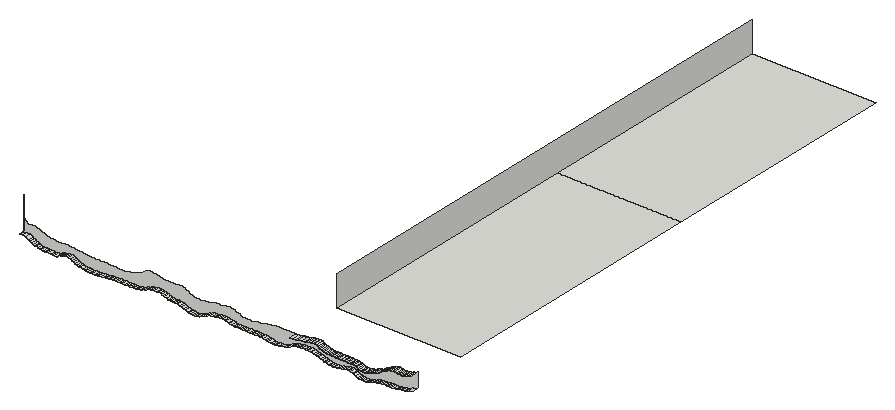
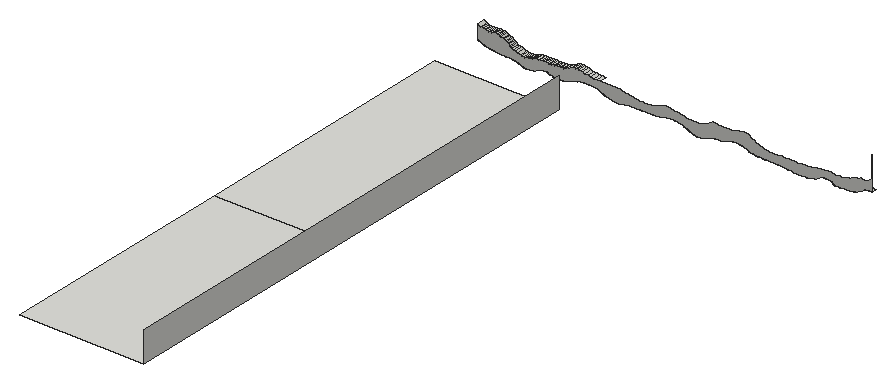
# SketchUp Ruby script. Lengths in inches.
U = 1.inch
M = Sketchup.active_model
def pt(a) = Geom::Point3d.new(a.map { |v| v * U })
def face(e, loops, mat)
  f = e.add_face(loops[0].map { |a| pt(a) })
  loops[1..].each { |l| e.add_face(l.map { |a| pt(a) }).erase! }
  f.material = f.back_material = mat if mat
  f
end
# faces: each face lists its corners as indices into pts; further lists are holes
def faces(e, pts, list, mat = nil) = list.each { |f| face(e, (f[0].is_a?(Array) ? f : [f]).map { |l| l.map { |i| pts[i] } }, mat) }
# xy, xz, yz: faces in a plane at the given z, y or x. An outline is a flat list of corners, or four numbers for a rectangle; further outlines are holes
def ring(l) = l.size == 4 ? [[l[0], l[1]], [l[2], l[1]], [l[2], l[3]], [l[0], l[3]]] : l.each_slice(2).to_a
def flat(e, list, mat, &to3) = list.each { |f| face(e, (f[0].is_a?(Array) ? f : [f]).map { |l| ring(l).map { |u, v| to3.(u, v) } }, mat) }
def xy(e, z, list, mat = nil) = flat(e, list, mat) { |x, y| [x, y, z] }
def xz(e, y, list, mat = nil) = flat(e, list, mat) { |x, z| [x, y, z] }
def yz(e, x, list, mat = nil) = flat(e, list, mat) { |y, z| [x, y, z] }
def lines(e, pts, list) = list.each { |a, b| e.add_line(pt(pts[a]), pt(pts[b])) }
# prism: a flat outline (further loops are holes) pulled along v
def prism(e, loops, v, mat = nil)
  f = face(e, loops, mat); d = Geom::Vector3d.new(v.map { |x| x * U })
  f.pushpull(f.normal.samedirection?(d) ? d.length : -d.length)
end
def box(e, o, s, mat = nil) = prism(e, [[o, [o[0] + s[0], o[1], o[2]], [o[0] + s[0], o[1] + s[1], o[2]], [o[0], o[1] + s[1], o[2]]]], [0, 0, s[2]], mat)
def at(x, y, z, deg = 0) = Geom::Transformation.translation(pt([x, y, z])) * Geom::Transformation.rotation(ORIGIN, Z_AXIS, deg.degrees)
def axes(o, x, y, z) = Geom::Transformation.new([*x, 0, *y, 0, *z, 0, *pt(o).to_a, 1])
def part(name) = M.definitions.add(name)
# library, detail: a bought-in or finely detailed component or shape, given as its bounding box
def library(name, o, s) = part(name).tap { |d| box(d.entities, o, s) }
def detail(e, o, s) = box(e.add_group.entities, o, s)
def put(e, d, t, mat = nil) = e.add_instance(d, t).tap { |i| i.material = mat if mat }
def group(e, t, mat = nil) = e.add_group.tap { |g| g.transformation = t; g.material = mat if mat }.entities
root = M.entities
xy(root,237.65,[[1160.83,2402.3,1161.52,2404.3],[1161.52,2402.3,1162.14,2404.3]])
xy(root,238.18,[[1254.78,2402.3,1255.46,2404.3]])
xy(root,238.33,[[1169.93,2402.3,1170.48,2404.3],[1170.48,2402.3,1171.16,2404.3]])
xy(root,238.34,[[1171.84,2402.3,1172.77,2404.3],[1172.77,2402.3,1173.26,2404.3],[1173.26,2402.3,1174.02,2404.3],[1174.02,2402.3,1174.65,2404.3],[1174.65,2402.3,1175.4,2404.3],
  [1175.4,2402.3,1176.02,2404.3],[1176.02,2402.3,1176.79,2404.3],[1176.79,2402.3,1177.41,2404.3]])
xy(root,238.62,[[1221.31,2402.3,1222.08,2404.3],[1222.08,2402.3,1222.71,2404.3],[1222.71,2402.3,1223.47,2404.3],[1223.47,2402.3,1224.09,2404.3],[1224.09,2402.3,1224.94,2404.3],
  [1224.94,2402.3,1225.58,2404.3],[1225.58,2402.3,1226.2,2404.3]])
xy(root,238.625,[[1219.89,2402.3,1220.75,2404.3]])
xy(root,238.89,[[1275.7,2402.3,1276.38,2404.3]])
xy(root,238.9,[[1277.14,2402.3,1277.76,2404.3],[1277.76,2402.3,1278.53,2404.3]])
xy(root,240.43,[[1243.98,2402.3,1244.55,2404.3]])
xy(root,241.52,[[1131.53,2402.3,1131.59,2404.3]])
xy(root,242.28,[[1261.8,2401.37,1262.3125,2404.3]])
xy(root,242.3,[[1260.04,2401.37,1260.71,2404.3]])
xy(root,242.33,[[1257.63,2401.37,1258.21,2404.3]])
xy(root,242.625,[[1237.14,2425.46,1285.6,2532.83],[1237.14,2532.83,1285.6,2628.15]])
xz(root,2404.3,[[1200.45,236.98,1199.84,237.01,1199.15,237.04,1198.39,237.11,1197.7,237.2,1197.17,237.33,1196.5,237.68,1195.5625,237.96,1195,238.28,1194.22,238.43,1193.44,238.78,1192.77,238.79,1192.23,238.8,1191.47,238.83,1190.72,238.875,1190.15,238.94,1189.57,239.04,1188.91,239.29,1188.33,239.53,1187.8,239.7,1187.11,239.92,1186.48,240.11,1185.7,240.27,1185.08,240.25,1184.375,240.23,1183.61,240.19,1182.9375,240.12,1182.28,240.03,1181.64,239.85,1181.09,239.52,1180.53,239.35,1179.94,239.18,1179.43,238.86,1178.74,238.72,1177.92,238.59,1177.41,238.34,1171.84,238.34,1171.16,238.33,1169.93,238.33,1169.21,238.32,1168.36,238.3,1167.73,238.28,1166.98,238.26,1166.35,238.15,1165.59,238.13,1165.04,238.1,1164.1875,237.98,1163.57,237.94,1162.81,237.89,1162.14,237.65,1160.83,237.65,1160.14,237.66,1159.39,237.67,1158.79,237.68,1158.18,237.71,1157.47,237.76,1156.78,237.82,1156.12,237.9,1155.18,238.21,1154.71,238.31,1153.8,238.43,1153.15,238.74,1152.57,239.11,1151.99,239.38,1151.53,239.71,1150.83,240.11,1150.14,240.09,1149.48,240.05,1148.89,239.99,1148.16,239.88,1147.61,239.69,1147.03,239.55,1146.47,238.9375,1145.94,238.77,1145.2,238.79,1144.33,238.8,1143.82,238.82,1142.78,238.92,1142.09,238.93,1141.39,238.94,1140.69,238.97,1140.01,239.03,1139.32,239.09,1138.54,239.19,1138.03,239.52,1137.47,239.64,1137.02,239.86,1136.23,240.2,1135.63,240.59,1135.09,240.85,1134.07,241.55,1132.8,241.69,1131.59,241.52,1131.59,246.2,1133.16,244.96,1134.55,244.9375,1135.8,244.92,1136.02,244.61,1136.58,244.54,1137.34,244.41,1138.01,244.11,1138.53,243.95,1139.19,243.79,1139.71,243.48,1140.35,243.3,1140.9375,243.14,1141.42,243.06,1142.14,242.85,1142.72,242.78,1143.53,242.73,1144.07,242.68,1144.74,242.51,1145.26,242.46,1145.8,242.58,1146.43,242.57,1147.06,242.81,1147.63,242.86,1148.19,242.89,1148.83,242.92,1149.26,242.625,1149.87,242.65,1150.42,242.62,1151.05,242.58,1151.61,242.57,1152.25,242.48,1152.91,242.38,1153.57,242.34,1154.24,242.24,1155.41,241.96,1156.18,241.89,1157,241.83,1157.6,241.78,1158.37,241.75,1158.82,241.74,1159.37,241.72,1160.63,241.7,1161.36,241.69,1162.03,241.68,1162.62,241.68,1163.11,241.67,1163.8125,241.74,1164.38,241.75,1166.38,241.75,1166.87,241.67,1167.4,241.66,1168.01,241.57,1168.55,241.53,1169.17,241.51,1169.72,241.49,1170.42,241.48,1171.08,241.47,1171.65,241.46,1172.36,241.6,1173.09,241.85,1173.76,241.91,1174.66,242.1,1175.43,242.46,1176.13,242.78,1176.9,242.97,1177.43,243.23,1177.83,243.48,1178.35,243.72,1178.6875,244.12,1179.16,244.39,1179.64,244.73,1180.125,244.87,1180.71,244.95,1181.39,245.01,1182.04,244.81,1182.61,244.7,1183.09,244.67,1183.7,244.55,1184.24,244.51,1184.7,244.25,1185.45,244.11,1186.01,244.04,1186.63,243.99,1187.35,243.95,1187.85,243.93,1188.54,243.91,1189.11,243.89,1189.81,243.88,1190.46,243.94,1191.1,243.95,1191.66,244.1,1192.29,244.13,1192.77,244.15,1193.29,244.17,1193.81,244.18,1194.41,243.8,1194.95,243.43,1195.56,243.09,1195.95,242.875,1196.45,242.68,1197.04,242.51,1197.55,242.21,1198.15,242.11,1198.83,241.96,1199.39,241.89,1199.85,241.85,1200.37,241.8125,1200.88,241.79,1201.46,241.78,1202.13,241.91,1202.6,241.93,1203.27,242.09,1204.04,242.2,1204.54,242.24,1205.15,242.42,1205.7,242.47,1206.45,242.71,1207.09,242.78,1207.57,242.82,1208.26,242.85,1208.96,242.87,1209.51,243.02,1210.13,243.05,1210.68,243.29,1211.36,243.35,1211.91,243.39,1212.51,243.42,1213.28,243.14,1213.85,242.9375,1214.4,242.65,1215.02,242.39,1215.78,242.14,1216.42,241.89,1216.91,241.78,1217.96,241.63,1218.73,241.56,1219.33,241.51,1219.78,241.48,1220.3,241.46,1221.17,241.51,1221.89,241.59,1222.83,241.82,1223.61,241.87,1224.375,241.98,1224.99,242.02,1225.64,242.19,1226.34,242.38,1226.83,242.4375,1227.35,242.48,1228.01,242.58,1228.54,242.61,1229.125,242.77,1229.58,242.95,1230.14,243.01,1230.65,243.05,1231.22,243.08,1231.875,243.09,1234.03,243.09,1234.6,243.08,1235.1875,243.07,1235.77,243.07,1236.43,243.0625,1237.04,243.05,1237.72,243.05,1238.99,243.1,1240.16,243.17,1241.3,243.4,1242.5625,243.52,1243.69,243.71,1244.59,243.99,1245.29,244.08,1245.99,244.21,1246.57,244.27,1247.11,244.3,1247.78,244.39,1248.375,244.19,1248.75,243.88,1249.23,243.59,1249.78,243.33,1250.33,243.22,1250.82,242.92,1251.3,242.75,1251.86,242.6,1252.42,242.52,1252.98,242.47,1253.5625,242.43,1254.14,242.4,1254.72,242.39,1255.3,242.37,1255.88,242.36,1256.47,242.35,1257.63,242.33,1258.21,242.33,1258.93,242.32,1259.4,242.3125,1260.04,242.3,1260.71,242.3,1261.16,242.29,1261.8,242.28,1262.3125,242.28,1262.94,242.2,1263.52,241.97,1264.09,241.84,1264.6,241.57,1265.02,241.33,1265.49,241.24,1266.02,241.17,1266.49,241.12,1267.09,241.09,1267.66,241.14,1268.3,241.35,1268.89,241.46,1269.83,241.85,1270.83,242.23,1271.39,242.42,1272.11,242.61,1272.625,242.91,1273,243.14,1273.54,243.52,1274.02,243.71,1274.35,244.02,1274.79,244.21,1275.38,244.57,1275.85,244.76,1276.47,245.125,1276.97,245.32,1277.45,245.41,1278,245.48,1278.49,245.59,1279.02,245.55,1279.63,245.35,1280.12,245.31,1280.67,245.27,1281.23,245.24,1281.79,245.22,1282.35,245.34,1282.98,245.42,1283.5625,245.52,1283.94,245.76,1284.41,245.9,1285.6,246.43,1285.6,240.89,1283.77,240.1,1283.21,239.96,1282.6875,239.81,1282,239.53,1281.45,239.49,1280.73,239.42,1279.93,239.28,1279.16,239.15,1278.53,238.9,1277.14,238.9,1276.38,238.89,1275.7,238.89,1275.02,238.88,1274.48,238.875,1273.72,238.86,1272.98,238.83,1272.41,238.8,1271.83,238.74,1271.17,238.6,1270.6,238.51,1270.07,238.33,1269.38,238.08,1268.7,237.84,1268.01,237.5625,1267.41,237.47,1266.73,237.4,1266,237.42,1265.43,237.45,1264.84,237.51,1264.24,237.59,1263.7,237.71,1262.87,238,1262.16,238.33,1261.61,238.57,1261.11,238.86,1260.59,238.96,1259.9,239.02,1259.22,239.125,1258.48,239.04,1257.91,238.66,1257.32,238.61,1256.66,238.55,1256.14,238.27,1255.46,238.18,1254.78,238.18,1254.11,238.11,1253.58,238.15,1252.76,238.19,1252.1875,238.26,1251.62,238.48,1250.96,238.56,1250.39,238.67,1249.87,239.01,1249.1875,239.18,1248.5625,239.5,1247.8,239.65,1247.1875,239.8,1246.43,239.96,1245.78,240.23,1245.2,240.27,1244.55,240.43,1243.98,240.43,1243.4,240.42,1242.875,240.41,1242.18,240.4,1241.49,240.37,1240.8,240.33,1240.12,240.27,1239.44,240.17,1238.82,239.97,1238.17,239.75,1237.43,239.375,1236.64,239.08,1235.76,238.72,1235.01,238.46,1233.79,238.14,1232.67,237.88,1232.02,237.87,1231.15,237.74,1230.44,237.79,1229.67,237.86,1229.04,238.15,1228.27,238.19,1227.65,238.25,1226.89,238.45,1226.2,238.62,1221.31,238.62,1220.75,238.625,1219.89,238.625,1219.2,238.63,1218.58,238.64,1217.8,238.65,1217.13,238.66,1216.44,238.6875,1215.77,238.73,1215.29,238.78,1214.41,238.93,1213.64,239.07,1213.09,239.16,1212.24,239.44,1211.57,239.56,1210.96,239.72,1210.23,239.7,1209.67,239.69,1209.08,239.65,1208.46,239.6,1207.97,239.54,1207.16,239.31,1206.16,239.22,1205.58,239.12,1204.9375,238.76,1204.3,238.51,1203.74,238.375,1203.3,238.02,1202.6,237.74,1201.98,237.43,1201.13,237.22],[1131.53,241.52,1131.59,254.5]])
yz(root,1237.14,[[2425.46,242.625,2628.15,254.5]])
p = [[1198.39,2404.3,237.11],[1199.15,2404.3,237.04],[1199.15,2402.3,237.04],[1198.39,2402.3,237.11],[1199.84,2404.3,237.01],[1199.84,2402.3,237.01],
  [1200.45,2404.3,236.98],[1200.45,2402.3,236.98],[1201.13,2404.3,237.22],[1201.13,2402.3,237.22],[1197.7,2404.3,237.2],[1197.7,2402.3,237.2],
  [1197.17,2404.3,237.33],[1197.17,2402.3,237.33],[1201.98,2404.3,237.43],[1201.98,2402.3,237.43],[1196.5,2404.3,237.68],[1196.5,2402.3,237.68],
  [1202.6,2404.3,237.74],[1202.6,2402.3,237.74],[1265.43,2404.3,237.45],[1266,2404.3,237.42],[1266,2402.3,237.42],[1265.43,2402.3,237.45],
  [1266.73,2404.3,237.4],[1266.73,2402.3,237.4],[1267.41,2404.3,237.47],[1267.41,2402.3,237.47],[1264.24,2404.3,237.59],[1264.84,2404.3,237.51],
  [1264.84,2402.3,237.51],[1264.24,2402.3,237.59],[1268.01,2404.3,237.5625],[1268.01,2402.3,237.5625],[1162.14,2404.3,237.65],[1162.81,2404.3,237.89],
  [1162.81,2402.3,237.89],[1162.14,2402.3,237.65],[1263.7,2404.3,237.71],[1263.7,2402.3,237.71],[1268.7,2404.3,237.84],[1268.7,2402.3,237.84],
  [1157.47,2404.3,237.76],[1158.18,2404.3,237.71],[1158.18,2402.3,237.71],[1157.47,2402.3,237.76],[1158.79,2404.3,237.68],[1158.79,2402.3,237.68],
  [1159.39,2404.3,237.67],[1159.39,2402.3,237.67],[1160.14,2404.3,237.66],[1160.14,2402.3,237.66],[1160.83,2404.3,237.65],[1160.83,2402.3,237.65],
  [1195.5625,2404.3,237.96],[1195.5625,2402.3,237.96],[1203.3,2404.3,238.02],[1203.3,2402.3,238.02],[1230.44,2404.3,237.79],[1231.15,2404.3,237.74],
  [1231.15,2402.3,237.74],[1230.44,2402.3,237.79],[1232.02,2404.3,237.87],[1232.02,2402.3,237.87],[1262.87,2404.3,238],[1262.87,2402.3,238],
  [1156.12,2404.3,237.9],[1156.78,2404.3,237.82],[1156.78,2402.3,237.82],[1156.12,2402.3,237.9],[1229.67,2404.3,237.86],[1229.67,2402.3,237.86],
  [1269.38,2404.3,238.08],[1269.38,2402.3,238.08],[1155.18,2404.3,238.21],[1155.18,2402.3,238.21],[1163.57,2404.3,237.94],[1163.57,2402.3,237.94],
  [1164.1875,2404.3,237.98],[1164.1875,2402.3,237.98],[1229.04,2404.3,238.15],[1229.04,2402.3,238.15],[1232.67,2404.3,237.88],[1232.67,2402.3,237.88],
  [1233.79,2404.3,238.14],[1233.79,2402.3,238.14],[1165.04,2404.3,238.1],[1165.04,2402.3,238.1],[1195,2404.3,238.28],[1195,2402.3,238.28],
  [1203.74,2404.3,238.375],[1203.74,2402.3,238.375],[1262.16,2404.3,238.33],[1262.16,2402.3,238.33],[1165.59,2404.3,238.13],[1165.59,2402.3,238.13],
  [1166.35,2404.3,238.15],[1166.35,2402.3,238.15],[1228.27,2404.3,238.19],[1228.27,2402.3,238.19],[1235.01,2404.3,238.46],[1235.01,2402.3,238.46],
  [1252.76,2404.3,238.19],[1253.58,2404.3,238.15],[1253.58,2402.3,238.15],[1252.76,2402.3,238.19],[1254.11,2404.3,238.11],[1254.11,2402.3,238.11],
  [1254.78,2404.3,238.18],[1254.78,2402.3,238.18],[1270.07,2404.3,238.33],[1270.07,2402.3,238.33],[1154.71,2404.3,238.31],[1154.71,2402.3,238.31],
  [1166.98,2404.3,238.26],[1166.98,2402.3,238.26],[1227.65,2404.3,238.25],[1227.65,2402.3,238.25],[1252.1875,2404.3,238.26],[1252.1875,2402.3,238.26],
  [1255.46,2404.3,238.18],[1256.14,2404.3,238.27],[1256.14,2402.3,238.27],[1255.46,2402.3,238.18],[1153.8,2404.3,238.43],[1153.8,2402.3,238.43],
  [1167.73,2404.3,238.28],[1167.73,2402.3,238.28],[1168.36,2404.3,238.3],[1168.36,2402.3,238.3],[1169.21,2404.3,238.32],[1169.21,2402.3,238.32],
  [1169.93,2404.3,238.33],[1169.93,2402.3,238.33],[1171.16,2404.3,238.33],[1171.84,2404.3,238.34],[1171.84,2402.3,238.34],[1171.16,2402.3,238.33],
  [1177.41,2404.3,238.34],[1177.92,2404.3,238.59],[1177.92,2402.3,238.59],[1177.41,2402.3,238.34],[1194.22,2404.3,238.43],[1194.22,2402.3,238.43],
  [1226.89,2404.3,238.45],[1226.89,2402.3,238.45],[1251.62,2404.3,238.48],[1251.62,2402.3,238.48],[1256.66,2404.3,238.55],[1256.66,2402.3,238.55],
  [1261.61,2404.3,238.57],[1261.61,2402.3,238.57],[1270.6,2404.3,238.51],[1270.6,2402.3,238.51],[1153.15,2404.3,238.74],[1153.15,2402.3,238.74],
  [1193.44,2404.3,238.78],[1193.44,2402.3,238.78],[1204.3,2404.3,238.51],[1204.3,2402.3,238.51],[1204.9375,2404.3,238.76],[1204.9375,2402.3,238.76],
  [1226.2,2404.3,238.62],[1226.2,2402.3,238.62],[1235.76,2404.3,238.72],[1235.76,2402.3,238.72],[1250.96,2404.3,238.56],[1250.96,2402.3,238.56],
  [1257.32,2404.3,238.61],[1257.32,2402.3,238.61],[1271.17,2404.3,238.6],[1271.17,2402.3,238.6],[1178.74,2404.3,238.72],[1178.74,2402.3,238.72],
  [1217.13,2404.3,238.66],[1217.8,2404.3,238.65],[1217.8,2402.3,238.65],[1217.13,2402.3,238.66],[1218.58,2404.3,238.64],[1218.58,2402.3,238.64],
  [1219.2,2404.3,238.63],[1219.2,2402.3,238.63],[1219.89,2404.3,238.625],[1219.89,2402.3,238.625],[1220.75,2404.3,238.625],[1221.31,2404.3,238.62],
  [1221.31,2402.3,238.62],[1220.75,2402.3,238.625],[1250.39,2404.3,238.67],[1250.39,2402.3,238.67],[1257.91,2404.3,238.66],[1257.91,2402.3,238.66],
  [1261.11,2404.3,238.86],[1261.11,2402.3,238.86],[1271.83,2404.3,238.74],[1271.83,2402.3,238.74],[1152.57,2404.3,239.11],[1152.57,2402.3,239.11],
  [1179.43,2404.3,238.86],[1179.43,2402.3,238.86],[1215.29,2404.3,238.78],[1215.77,2404.3,238.73],[1215.77,2402.3,238.73],[1215.29,2402.3,238.78],
  [1216.44,2404.3,238.6875],[1216.44,2402.3,238.6875],[1236.64,2404.3,239.08],[1236.64,2402.3,239.08],[1249.87,2404.3,239.01],[1249.87,2402.3,239.01],
  [1258.48,2404.3,239.04],[1258.48,2402.3,239.04],[1272.41,2404.3,238.8],[1272.41,2402.3,238.8],[1142.78,2404.3,238.92],[1143.82,2404.3,238.82],
  [1143.82,2402.3,238.82],[1142.78,2402.3,238.92],[1144.33,2404.3,238.8],[1144.33,2402.3,238.8],[1145.2,2404.3,238.79],[1145.2,2402.3,238.79],
  [1145.94,2404.3,238.77],[1145.94,2402.3,238.77],[1146.47,2404.3,238.9375],[1146.47,2402.3,238.9375],[1190.72,2404.3,238.875],[1191.47,2404.3,238.83],
  [1191.47,2402.3,238.83],[1190.72,2402.3,238.875],[1192.23,2404.3,238.8],[1192.23,2402.3,238.8],[1192.77,2404.3,238.79],[1192.77,2402.3,238.79],
  [1205.58,2404.3,239.12],[1205.58,2402.3,239.12],[1214.41,2404.3,238.93],[1214.41,2402.3,238.93],[1272.98,2404.3,238.83],[1272.98,2402.3,238.83],
  [1273.72,2404.3,238.86],[1273.72,2402.3,238.86],[1140.69,2404.3,238.97],[1141.39,2404.3,238.94],[1141.39,2402.3,238.94],[1140.69,2402.3,238.97],
  [1142.09,2404.3,238.93],[1142.09,2402.3,238.93],[1147.03,2404.3,239.55],[1147.03,2402.3,239.55],[1179.94,2404.3,239.18],[1179.94,2402.3,239.18],
  [1189.57,2404.3,239.04],[1190.15,2404.3,238.94],[1190.15,2402.3,238.94],[1189.57,2402.3,239.04],[1213.64,2404.3,239.07],[1213.64,2402.3,239.07],
  [1260.59,2404.3,238.96],[1260.59,2402.3,238.96],[1274.48,2404.3,238.875],[1274.48,2402.3,238.875],[1275.02,2404.3,238.88],[1275.02,2402.3,238.88],
  [1275.7,2404.3,238.89],[1275.7,2402.3,238.89],[1276.38,2404.3,238.89],[1277.14,2404.3,238.9],[1277.14,2402.3,238.9],[1276.38,2402.3,238.89],
  [1278.53,2404.3,238.9],[1279.16,2404.3,239.15],[1279.16,2402.3,239.15],[1278.53,2402.3,238.9],[1139.32,2404.3,239.09],[1140.01,2404.3,239.03],
  [1140.01,2402.3,239.03],[1139.32,2402.3,239.09],[1188.91,2404.3,239.29],[1188.91,2402.3,239.29],[1249.1875,2404.3,239.18],[1249.1875,2402.3,239.18],
  [1259.22,2404.3,239.125],[1259.22,2402.3,239.125],[1259.9,2404.3,239.02],[1259.9,2402.3,239.02],[1138.54,2404.3,239.19],[1138.54,2402.3,239.19],
  [1151.99,2404.3,239.38],[1151.99,2402.3,239.38],[1206.16,2404.3,239.22],[1206.16,2402.3,239.22],[1213.09,2404.3,239.16],[1213.09,2402.3,239.16],
  [1237.43,2404.3,239.375],[1237.43,2402.3,239.375],[1138.03,2404.3,239.52],[1138.03,2402.3,239.52],[1180.53,2404.3,239.35],[1180.53,2402.3,239.35],
  [1207.16,2404.3,239.31],[1207.16,2402.3,239.31],[1212.24,2404.3,239.44],[1212.24,2402.3,239.44],[1248.5625,2404.3,239.5],[1248.5625,2402.3,239.5],
  [1279.93,2404.3,239.28],[1279.93,2402.3,239.28],[1188.33,2404.3,239.53],[1188.33,2402.3,239.53],[1207.97,2404.3,239.54],[1207.97,2402.3,239.54],
  [1280.73,2404.3,239.42],[1280.73,2402.3,239.42],[1151.53,2404.3,239.71],[1151.53,2402.3,239.71],[1181.09,2404.3,239.52],[1181.09,2402.3,239.52],
  [1211.57,2404.3,239.56],[1211.57,2402.3,239.56],[1238.17,2404.3,239.75],[1238.17,2402.3,239.75],[1281.45,2404.3,239.49],[1281.45,2402.3,239.49],
  [1137.47,2404.3,239.64],[1137.47,2402.3,239.64],[1181.64,2404.3,239.85],[1181.64,2402.3,239.85],[1187.8,2404.3,239.7],[1187.8,2402.3,239.7],
  [1208.46,2404.3,239.6],[1208.46,2402.3,239.6],[1247.8,2404.3,239.65],[1247.8,2402.3,239.65],[1282,2404.3,239.53],[1282,2402.3,239.53],
  [1282.6875,2404.3,239.81],[1282.6875,2402.3,239.81],[1137.02,2404.3,239.86],[1137.02,2402.3,239.86],[1147.61,2404.3,239.69],[1147.61,2402.3,239.69],
  [1209.08,2404.3,239.65],[1209.08,2402.3,239.65],[1209.67,2404.3,239.69],[1209.67,2402.3,239.69],[1210.96,2404.3,239.72],[1210.96,2402.3,239.72],
  [1148.16,2404.3,239.88],[1148.16,2402.3,239.88],[1150.83,2404.3,240.11],[1150.83,2402.3,240.11],[1187.11,2404.3,239.92],[1187.11,2402.3,239.92],
  [1210.23,2404.3,239.7],[1210.23,2402.3,239.7],[1238.82,2404.3,239.97],[1238.82,2402.3,239.97],[1247.1875,2404.3,239.8],[1247.1875,2402.3,239.8],
  [1182.28,2404.3,240.03],[1182.28,2402.3,240.03],[1246.43,2404.3,239.96],[1246.43,2402.3,239.96],[1283.21,2404.3,239.96],[1283.21,2402.3,239.96],
  [1136.23,2404.3,240.2],[1136.23,2402.3,240.2],[1148.89,2404.3,239.99],[1148.89,2402.3,239.99],[1186.48,2404.3,240.11],[1186.48,2402.3,240.11],
  [1149.48,2404.3,240.05],[1149.48,2402.3,240.05],[1150.14,2404.3,240.09],[1150.14,2402.3,240.09],[1182.9375,2404.3,240.12],[1182.9375,2402.3,240.12],
  [1239.44,2404.3,240.17],[1239.44,2402.3,240.17],[1245.78,2404.3,240.23],[1245.78,2402.3,240.23],[1283.77,2404.3,240.1],[1283.77,2402.3,240.1],
  [1183.61,2404.3,240.19],[1183.61,2402.3,240.19],[1185.7,2404.3,240.27],[1185.7,2402.3,240.27],[1285.6,2404.3,240.89],[1285.6,2402.3,240.89],
  [1135.63,2404.3,240.59],[1135.63,2402.3,240.59],[1184.375,2404.3,240.23],[1184.375,2402.3,240.23],[1185.08,2404.3,240.25],[1185.08,2402.3,240.25],
  [1240.12,2404.3,240.27],[1240.12,2402.3,240.27],[1245.2,2404.3,240.27],[1245.2,2402.3,240.27],[1240.8,2404.3,240.33],[1240.8,2402.3,240.33],
  [1241.49,2404.3,240.37],[1241.49,2402.3,240.37],[1244.55,2404.3,240.43],[1244.55,2402.3,240.43],[1242.18,2404.3,240.4],[1242.18,2402.3,240.4],
  [1242.875,2404.3,240.41],[1242.875,2402.3,240.41],[1243.4,2404.3,240.42],[1243.4,2402.3,240.42],[1243.98,2404.3,240.43],[1243.98,2402.3,240.43],
  [1135.09,2404.3,240.85],[1135.09,2402.3,240.85],[1134.07,2404.3,241.55],[1134.07,2402.3,241.55],[1266.02,2404.3,241.17],[1266.49,2404.3,241.12],
  [1266.49,2401.37,241.12],[1266.02,2401.37,241.17],[1267.09,2404.3,241.09],[1267.09,2401.37,241.09],[1267.66,2404.3,241.14],[1267.66,2401.37,241.14],
  [1268.3,2404.3,241.35],[1268.3,2401.37,241.35],[1265.02,2404.3,241.33],[1265.49,2404.3,241.24],[1265.49,2401.37,241.24],[1265.02,2401.37,241.33],
  [1264.6,2404.3,241.57],[1264.6,2401.37,241.57],[1268.89,2404.3,241.46],[1268.89,2401.37,241.46],[1269.83,2404.3,241.85],[1269.83,2401.37,241.85],
  [1131.59,2404.3,241.52],[1132.8,2404.3,241.69],[1132.8,2402.3,241.69],[1131.59,2402.3,241.52],[1264.09,2404.3,241.84],[1264.09,2401.37,241.84],
  [1263.52,2404.3,241.97],[1263.52,2401.37,241.97],[1270.83,2404.3,242.23],[1270.83,2401.37,242.23],[1262.94,2404.3,242.2],[1262.94,2401.37,242.2],
  [1262.3125,2404.3,242.28],[1262.3125,2401.37,242.28],[1271.39,2404.3,242.42],[1271.39,2401.37,242.42],[1256.47,2404.3,242.35],[1257.05,2404.3,242.34],
  [1257.05,2401.37,242.34],[1256.47,2401.37,242.35],[1257.63,2404.3,242.33],[1257.63,2401.37,242.33],[1258.21,2404.3,242.33],[1258.93,2404.3,242.32],
  [1258.93,2401.37,242.32],[1258.21,2401.37,242.33],[1259.4,2404.3,242.3125],[1259.4,2401.37,242.3125],[1260.04,2404.3,242.3],[1260.04,2401.37,242.3],
  [1260.71,2404.3,242.3],[1261.16,2404.3,242.29],[1261.16,2401.37,242.29],[1260.71,2401.37,242.3],[1261.8,2404.3,242.28],[1261.8,2401.37,242.28],
  [1252.98,2404.3,242.47],[1253.5625,2404.3,242.43],[1253.5625,2401.37,242.43],[1252.98,2401.37,242.47],[1254.14,2404.3,242.4],[1254.14,2401.37,242.4],
  [1254.72,2404.3,242.39],[1254.72,2401.37,242.39],[1255.3,2404.3,242.37],[1255.3,2401.37,242.37],[1255.88,2404.3,242.36],[1255.88,2401.37,242.36],
  [1272.11,2404.3,242.61],[1272.11,2401.37,242.61],[1251.86,2404.3,242.6],[1252.42,2404.3,242.52],[1252.42,2401.37,242.52],[1251.86,2401.37,242.6],
  [1251.3,2404.3,242.75],[1251.3,2401.37,242.75],[1272.625,2404.3,242.91],[1272.625,2401.37,242.91],[1250.82,2404.3,242.92],[1250.82,2401.37,242.92],
  [1250.33,2404.3,243.22],[1250.33,2401.37,243.22],[1273,2404.3,243.14],[1273,2401.37,243.14],[1237.72,2404.3,243.05],[1238.99,2404.3,243.1],
  [1238.99,2401.37,243.1],[1237.72,2401.37,243.05],[1240.16,2404.3,243.17],[1240.16,2401.37,243.17],[1273.54,2404.3,243.52],[1273.54,2401.37,243.52],
  [1241.3,2404.3,243.4],[1241.3,2401.37,243.4],[1249.78,2404.3,243.33],[1249.78,2401.37,243.33],[1249.23,2404.3,243.59],[1249.23,2401.37,243.59],
  [1242.5625,2404.3,243.52],[1242.5625,2401.37,243.52],[1243.69,2404.3,243.71],[1243.69,2401.37,243.71],[1274.02,2404.3,243.71],[1274.02,2401.37,243.71],
  [1248.75,2404.3,243.88],[1248.75,2401.37,243.88],[1244.59,2404.3,243.99],[1244.59,2401.37,243.99],[1274.35,2404.3,244.02],[1274.35,2401.37,244.02],
  [1248.375,2404.3,244.19],[1248.375,2401.37,244.19],[1245.29,2404.3,244.08],[1245.29,2401.37,244.08],[1274.79,2404.3,244.21],[1274.79,2401.37,244.21],
  [1245.99,2404.3,244.21],[1245.99,2401.37,244.21],[1246.57,2404.3,244.27],[1246.57,2401.37,244.27],[1247.78,2404.3,244.39],[1247.78,2401.37,244.39],
  [1275.38,2404.3,244.57],[1275.38,2401.37,244.57],[1247.11,2404.3,244.3],[1247.11,2401.37,244.3],[1275.85,2404.3,244.76],[1275.85,2401.37,244.76],
  [1276.47,2404.3,245.125],[1276.47,2401.37,245.125],[1276.97,2404.3,245.32],[1276.97,2401.37,245.32],[1280.67,2404.3,245.27],[1281.23,2404.3,245.24],
  [1281.23,2401.37,245.24],[1280.67,2401.37,245.27],[1281.79,2404.3,245.22],[1281.79,2401.37,245.22],[1282.35,2404.3,245.34],[1282.35,2401.37,245.34],
  [1277.45,2404.3,245.41],[1277.45,2401.37,245.41],[1279.02,2404.3,245.55],[1279.63,2404.3,245.35],[1279.63,2401.37,245.35],[1279.02,2401.37,245.55],
  [1280.12,2404.3,245.31],[1280.12,2401.37,245.31],[1282.98,2404.3,245.42],[1282.98,2401.37,245.42],[1278,2404.3,245.48],[1278,2401.37,245.48],
  [1283.5625,2404.3,245.52],[1283.5625,2401.37,245.52],[1278.49,2404.3,245.59],[1278.49,2401.37,245.59],[1283.94,2404.3,245.76],[1283.94,2401.37,245.76],
  [1284.41,2404.3,245.9],[1284.41,2401.37,245.9],[1285.6,2404.3,246.43],[1285.6,2401.37,246.43]]
faces(root,p,[[0,1,2,3],[1,4,5,2],[4,6,7,5],[6,8,9,7],[10,0,3,11],[12,10,11,13],[8,14,15,9],[16,12,13,17],
  [14,18,19,15],[20,21,22,23],[21,24,25,22],[24,26,27,25],[28,29,30,31],[29,20,23,30],[26,32,33,27],[34,35,36,37],
  [38,28,31,39],[32,40,41,33],[42,43,44,45],[43,46,47,44],[46,48,49,47],[48,50,51,49],[50,52,53,51],[54,16,17,55],
  [18,56,57,19],[58,59,60,61],[59,62,63,60],[64,38,39,65],[66,67,68,69],[67,42,45,68],[70,58,61,71],[40,72,73,41],
  [74,66,69,75],[35,76,77,36],[76,78,79,77],[80,70,71,81],[62,82,83,63],[82,84,85,83],[78,86,87,79],[88,54,55,89],
  [56,90,91,57],[92,64,65,93],[86,94,95,87],[94,96,97,95],[98,80,81,99],[84,100,101,85],[102,103,104,105],[103,106,107,104],
  [106,108,109,107],[72,110,111,73],[112,74,75,113],[96,114,115,97],[116,98,99,117],[118,102,105,119],[120,121,122,123],[124,112,113,125],
  [114,126,127,115],[126,128,129,127],[128,130,131,129],[130,132,133,131],[134,135,136,137],[138,139,140,141],[142,88,89,143],[144,116,117,145],
  [146,118,119,147],[121,148,149,122],[150,92,93,151],[110,152,153,111],[154,124,125,155],[156,142,143,157],[90,158,159,91],[158,160,161,159],
  [162,144,145,163],[100,164,165,101],[166,146,147,167],[148,168,169,149],[152,170,171,153],[139,172,173,140],[174,175,176,177],[175,178,179,176],
  [178,180,181,179],[180,182,183,181],[184,185,186,187],[188,166,167,189],[168,190,191,169],[192,150,151,193],[170,194,195,171],[196,154,155,197],
  [172,198,199,173],[200,201,202,203],[201,204,205,202],[204,174,177,205],[164,206,207,165],[208,188,189,209],[190,210,211,191],[194,212,213,195],
  [214,215,216,217],[215,218,219,216],[218,220,221,219],[220,222,223,221],[222,224,225,223],[226,227,228,229],[227,230,231,228],[230,232,233,231],
  [232,156,157,233],[160,234,235,161],[236,200,203,237],[212,238,239,213],[238,240,241,239],[242,243,244,245],[243,246,247,244],[246,214,217,247],
  [224,248,249,225],[198,250,251,199],[252,253,254,255],[253,226,229,254],[256,236,237,257],[258,192,193,259],[240,260,261,241],[260,262,263,261],
  [262,264,265,263],[266,267,268,269],[270,271,272,273],[274,275,276,277],[275,242,245,276],[278,252,255,279],[280,208,209,281],[210,282,283,211],
  [282,284,285,283],[284,258,259,285],[286,274,277,287],[288,196,197,289],[234,290,291,235],[292,256,257,293],[206,294,295,207],[296,286,287,297],
  [250,298,299,251],[290,300,301,291],[302,292,293,303],[304,280,281,305],[271,306,307,272],[308,278,279,309],[300,310,311,301],[306,312,313,307],
  [314,288,289,315],[298,316,317,299],[318,302,303,319],[294,320,321,295],[312,322,323,313],[324,296,297,325],[316,326,327,317],[328,308,309,329],
  [310,330,331,311],[332,304,305,333],[322,334,335,323],[334,336,337,335],[338,324,325,339],[248,340,341,249],[330,342,343,331],[342,344,345,343],
  [346,318,319,347],[340,348,349,341],[350,314,315,351],[352,328,329,353],[344,354,355,345],[354,346,347,355],[320,356,357,321],[358,332,333,359],
  [326,360,361,327],[362,358,359,363],[336,364,365,337],[366,338,339,367],[348,368,369,349],[370,352,353,371],[368,372,373,369],[372,374,375,373],
  [360,376,377,361],[356,378,379,357],[380,362,363,381],[364,382,383,365],[374,350,351,375],[376,384,385,377],[386,370,371,387],[382,388,389,383],
  [390,366,367,391],[384,392,393,385],[392,394,395,393],[378,396,397,379],[398,380,381,399],[394,386,387,395],[396,400,401,397],[400,402,403,401],
  [404,398,399,405],[402,406,407,403],[406,408,409,407],[408,410,411,409],[410,412,413,411],[414,390,391,415],[416,414,415,417],[418,419,420,421],
  [419,422,423,420],[422,424,425,423],[424,426,427,425],[428,429,430,431],[429,418,421,430],[432,428,431,433],[426,434,435,427],[434,436,437,435],
  [438,439,440,441],[442,432,433,443],[439,416,417,440],[444,442,443,445],[436,446,447,437],[448,444,445,449],[450,448,449,451],[446,452,453,447],
  [454,455,456,457],[455,458,459,456],[460,461,462,463],[461,464,465,462],[464,466,467,465],[468,469,470,471],[469,472,473,470],[474,475,476,477],
  [475,478,479,476],[478,480,481,479],[480,482,483,481],[482,484,485,483],[484,454,457,485],[452,486,487,453],[488,489,490,491],[489,474,477,490],
  [492,488,491,493],[486,494,495,487],[496,492,493,497],[498,496,497,499],[494,500,501,495],[502,503,504,505],[503,506,507,504],[500,508,509,501],
  [506,510,511,507],[512,498,499,513],[514,512,513,515],[510,516,517,511],[516,518,519,517],[508,520,521,509],[522,514,515,523],[518,524,525,519],
  [520,526,527,521],[528,522,523,529],[524,530,531,525],[526,532,533,527],[530,534,535,531],[534,536,537,535],[538,528,529,539],[532,540,541,533],
  [536,542,543,537],[542,538,539,543],[540,544,545,541],[544,546,547,545],[546,548,549,547],[550,551,552,553],[551,554,555,552],[554,556,557,555],
  [548,558,559,549],[560,561,562,563],[561,564,565,562],[564,550,553,565],[556,566,567,557],[558,568,569,559],[566,570,571,567],[568,572,573,569],
  [570,574,575,571],[572,560,563,573],[574,576,577,575],[576,578,579,577]])
